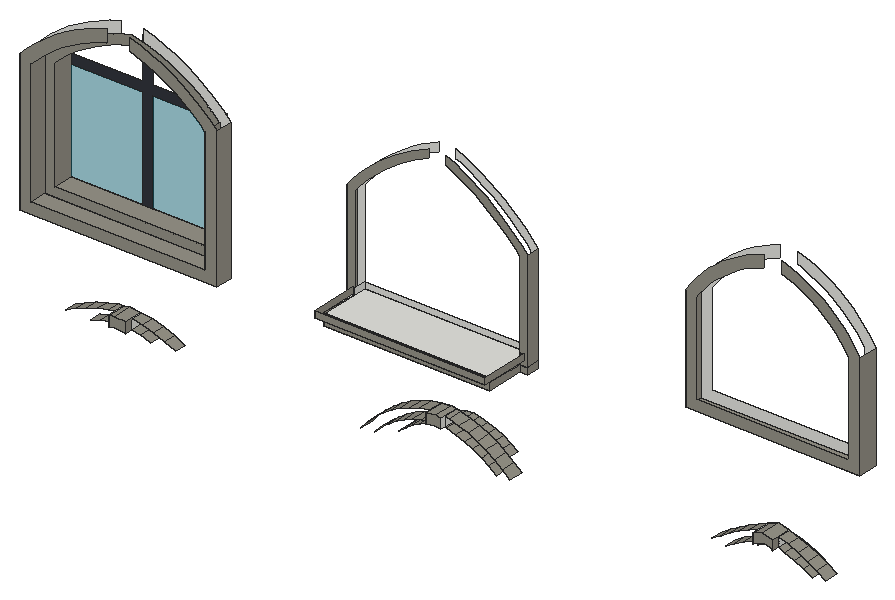
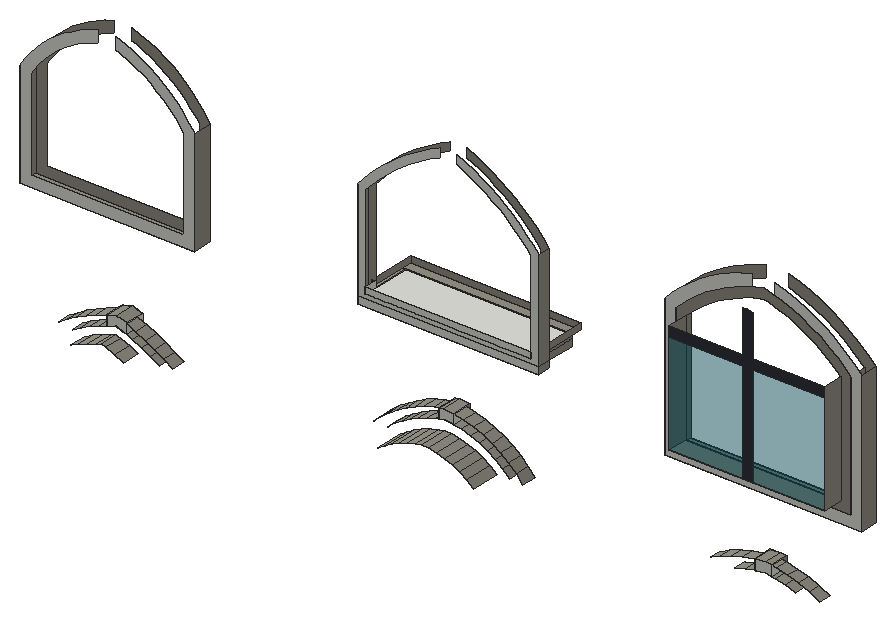
# SketchUp Ruby script. Lengths in inches.
U = 1.inch
M = Sketchup.active_model
def pt(a) = Geom::Point3d.new(a.map { |v| v * U })
def face(e, loops, mat)
  f = e.add_face(loops[0].map { |a| pt(a) })
  loops[1..].each { |l| e.add_face(l.map { |a| pt(a) }).erase! }
  f.material = f.back_material = mat if mat
  f
end
# faces: each face lists its corners as indices into pts; further lists are holes
def faces(e, pts, list, mat = nil) = list.each { |f| face(e, (f[0].is_a?(Array) ? f : [f]).map { |l| l.map { |i| pts[i] } }, mat) }
# xy, xz, yz: faces in a plane at the given z, y or x. An outline is a flat list of corners, or four numbers for a rectangle; further outlines are holes
def ring(l) = l.size == 4 ? [[l[0], l[1]], [l[2], l[1]], [l[2], l[3]], [l[0], l[3]]] : l.each_slice(2).to_a
def flat(e, list, mat, &to3) = list.each { |f| face(e, (f[0].is_a?(Array) ? f : [f]).map { |l| ring(l).map { |u, v| to3.(u, v) } }, mat) }
def xy(e, z, list, mat = nil) = flat(e, list, mat) { |x, y| [x, y, z] }
def xz(e, y, list, mat = nil) = flat(e, list, mat) { |x, z| [x, y, z] }
def yz(e, x, list, mat = nil) = flat(e, list, mat) { |y, z| [x, y, z] }
def lines(e, pts, list) = list.each { |a, b| e.add_line(pt(pts[a]), pt(pts[b])) }
# prism: a flat outline (further loops are holes) pulled along v
def prism(e, loops, v, mat = nil)
  f = face(e, loops, mat); d = Geom::Vector3d.new(v.map { |x| x * U })
  f.pushpull(f.normal.samedirection?(d) ? d.length : -d.length)
end
def box(e, o, s, mat = nil) = prism(e, [[o, [o[0] + s[0], o[1], o[2]], [o[0] + s[0], o[1] + s[1], o[2]], [o[0], o[1] + s[1], o[2]]]], [0, 0, s[2]], mat)
def at(x, y, z, deg = 0) = Geom::Transformation.translation(pt([x, y, z])) * Geom::Transformation.rotation(ORIGIN, Z_AXIS, deg.degrees)
def axes(o, x, y, z) = Geom::Transformation.new([*x, 0, *y, 0, *z, 0, *pt(o).to_a, 1])
def part(name) = M.definitions.add(name)
# library, detail: a bought-in or finely detailed component or shape, given as its bounding box
def library(name, o, s) = part(name).tap { |d| box(d.entities, o, s) }
def detail(e, o, s) = box(e.add_group.entities, o, s)
def put(e, d, t, mat = nil) = e.add_instance(d, t).tap { |i| i.material = mat if mat }
def group(e, t, mat = nil) = e.add_group.tap { |g| g.transformation = t; g.material = mat if mat }.entities
root = M.entities
M.materials.add("[Formica Graystone]").color = [149, 146, 135]
M.materials.add("[Formica Laminate Dark]").color = [50, 53, 60]
M.materials.add("[Translucent Glass Tinted]").color = [4, 106, 127]
M.materials["[Translucent Glass Tinted]"].alpha = 0.48
xy(root,431.0625,[[55.73,135.41,152.02,144.04]],"[Formica Graystone]")
xy(root,436.63,[[61.3,135.41,146.45,144.04]],"[Formica Graystone]")
xy(root,441.07,[[65.73,144.04,142.02,154.22]],"[Formica Graystone]")
xy(root,444.43,[[217.65,119.16,217.65,137.66,213.87,137.66,213.87,144.04,302.49,144.04,302.49,137.66,298.71,137.66,298.71,119.16]],"[Formica Graystone]")
xy(root,447.8,[[217.65,119.16,298.71,119.16,298.71,137.66,302.49,137.66,302.49,144.04,213.87,144.04,213.87,137.66,217.65,137.66]])
xy(root,449.51,[[370.76,148.68,456.27,158.3]],"[Formica Graystone]")
xy(root,449.83,[[216.84,119.16,217.65,137.66],[217.65,119.16,298.71,144.04]])
xy(root,449.83,[[216.84,114.16,300.34,119.16],[298.71,119.16,300.34,137.66]],"[Formica Graystone]")
xz(root,114.16,[[216.84,449.83,300.34,452.9]],"[Formica Graystone]")
xz(root,119.16,[[217.65,444.43,298.71,447.8],[217.65,447.8,298.71,449.83]],"[Formica Graystone]")
xz(root,134.29,[[262.44,408.08,262.44,412.87,260.05,413.37,255.1,412.87,255.1,408.09,255.79,408.23,259.8,408.63]],"[Formica Graystone]")
xz(root,134.6,[[108.25,395.78,108.25,400.8125,102.66,401.34,99.89,400.96,99.89,395.97,102.76,396.35,107.57,395.9]],"[Formica Graystone]")
xz(root,135.41,[[55.73,431.0625,152.02,431.0625,152.02,499.53,148.09,503.55,143.91,507.3,139.5,510.79,134.89,513.99,130.08,516.9,125.1,519.51,119.96,521.79,114.7,523.75,109.32,525.375,109.32,519.5625,112.92,518.47,117.86,516.64,122.67,514.49,127.35,512.05,131.85,509.32,136.18,506.32,140.32,503.05,144.23,499.52,146.45,497.26,146.45,436.63,61.3,436.63,61.3,497.1875,63.52,499.43,67.45,502.9375,71.59,506.2,75.92,509.2,80.43,511.9375,85.1,514.39,89.91,516.55,94.84,518.41,98.39,519.51,98.39,525.34,93.03,523.68,87.78,521.7,82.66,519.4,77.69,516.79,72.89,513.875,68.28,510.68,63.87,507.2,59.68,503.46,55.73,499.48]],"[Formica Graystone]")
xz(root,137.66,[[216.84,449.83,217.65,452.9],[298.71,449.83,300.34,452.9]])
xz(root,137.66,[[213.87,444.43,217.65,447.8],[298.71,444.43,302.49,447.8],[213.87,447.8,217.65,447.8,217.65,449.83,216.84,449.83,216.84,452.9,217.65,452.9,217.65,495.41,219.67,497.78,222.68,501.01,225.83,504.11,229.125,507.06,232.54,509.86,236.08,512.5,239.74,514.99,243.5,517.3,247.37,519.45,251.32,521.42,253.91,522.5625,253.91,526.7,249.71,524.84,245.6,522.8,241.59,520.57,237.68,518.16,233.89,515.59,230.21,512.84,226.66,509.93,223.25,506.87,219.97,503.65,216.84,500.3,213.87,496.8],[298.71,447.8,302.49,447.8,302.49,496.8,299.44,500.21,296.25,503.5,292.9375,506.65,289.49,509.67,285.93,512.55,282.26,515.28,278.48,517.86,274.59,520.28,270.62,522.55,266.55,524.66,262.4,526.6,262.4,522.42,264.88,521.26,268.81,519.23,272.65,517.04,276.41,514.69,280.0625,512.2,283.61,509.56,287.06,506.78,290.38,503.86,293.59,500.81,296.67,497.63,298.71,495.36,298.71,452.9,300.34,452.9,300.34,449.83,298.71,449.83]],"[Formica Graystone]")
xz(root,144.04,[[108.25,395.78,107.57,395.9,102.76,396.35,99.89,395.97,99.89,400.96,102.66,401.34,108.25,400.8125],[262.44,408.08,259.8,408.63,255.79,408.23,255.1,408.09,255.1,412.87,260.05,413.37,262.44,412.87],[55.73,431.0625,55.73,499.48,59.68,503.46,63.87,507.2,68.28,510.68,72.89,513.875,77.69,516.79,82.66,519.4,87.78,521.7,93.03,523.68,98.39,525.34,98.39,519.51,94.84,518.41,89.91,516.55,85.1,514.39,80.43,511.9375,75.92,509.2,71.59,506.2,67.45,502.9375,63.52,499.43,61.3,497.1875,61.3,436.63,146.45,436.63,146.45,497.26,144.23,499.52,140.32,503.05,136.18,506.32,131.85,509.32,127.35,512.05,122.67,514.49,117.86,516.64,112.92,518.47,109.32,519.5625,109.32,525.375,114.7,523.75,119.96,521.79,125.1,519.51,130.08,516.9,134.89,513.99,139.5,510.79,143.91,507.3,148.09,503.55,152.02,499.53,152.02,431.0625],[213.87,444.43,302.49,447.8],[213.87,447.8,213.87,496.8,216.84,500.3,219.97,503.65,223.25,506.87,226.66,509.93,230.21,512.84,233.89,515.59,237.68,518.16,241.59,520.57,245.6,522.8,249.71,524.84,253.91,526.7,253.91,522.5625,251.32,521.42,247.37,519.45,243.5,517.3,239.74,514.99,236.08,512.5,232.54,509.86,229.125,507.06,225.83,504.11,222.68,501.01,219.67,497.78,217.65,495.41,217.65,449.83,298.71,449.83,298.71,495.36,296.67,497.63,293.59,500.81,290.38,503.86,287.06,506.78,283.61,509.56,280.0625,512.2,276.41,514.69,272.65,517.04,268.81,519.23,264.88,521.26,262.4,522.42,262.4,526.6,266.55,524.66,270.62,522.55,274.59,520.28,278.48,517.86,282.26,515.28,285.93,512.55,289.49,509.67,292.9375,506.65,296.25,503.5,299.44,500.21,302.49,496.8,302.49,447.8],
  [217.65,449.83,298.71,452.9]])
xz(root,144.04,[[[61.3,436.63,146.45,436.63,146.45,497.26,144.23,499.52,140.32,503.05,136.18,506.32,131.85,509.32,127.35,512.05,122.67,514.49,117.86,516.64,112.92,518.47,109.32,519.5625,107.875,520,103.87,520.9375,99.875,519.97,98.39,519.51,94.84,518.41,89.91,516.55,85.1,514.39,80.43,511.9375,75.92,509.2,71.59,506.2,67.45,502.9375,63.52,499.43,61.3,497.1875],[65.73,441.07,65.73,495.36,66.57,496.21,70.3,499.54,74.23,502.63,78.34,505.48,82.61,508.07,87.04,510.4,91.6,512.45,96.28,514.21,101.05,515.6875,103.89,516.375,106.73,515.71,111.5,514.27,116.18,512.53,120.74,510.5,125.17,508.18,129.4375,505.6,133.54,502.75,137.45,499.65,141.16,496.32,142.02,495.45,142.02,441.07]]],"[Formica Graystone]")
xz(root,148.55,[[404.07,401.49,405.7,402.17,409.0625,403.41,412.52,402.41,413.875,401.94,413.875,406.64,408.9,408.09,404.07,406.31]],"[Formica Graystone]")
xz(root,148.68,[[370.76,449.51,456.27,449.51,456.27,500.95,453.8,504.68,451.07,508.24,448.12,511.6,444.94,514.76,441.56,517.7,437.99,520.4,434.24,522.86,430.34,525.06,426.29,526.99,422.13,528.65,417.87,530.02,417.87,524.45,420.34,523.66,424.17,522.13,427.89,520.36,431.48,518.33,434.93,516.07,438.22,513.58,441.33,510.88,444.25,507.97,446.98,504.875,449.48,501.6,450.98,499.35,450.98,454.81,376.06,454.81,376.06,499.26,377.57,501.39,380.16,504.61,382.95,507.66,385.92,510.53,389.0625,513.22,392.36,515.7,395.8125,517.98,399.4,520.04,403.1,521.87,406.91,523.47,409.22,524.28,409.22,529.89,405.01,528.42,400.9,526.69,396.9,524.71,393.03,522.49,389.31,520.03,385.74,517.35,382.35,514.45,379.15,511.35,376.14,508.06,373.34,504.58,370.76,500.95]],"[Formica Graystone]")
xz(root,154.22,[[101.05,441.07,105.93,441.07,105.93,490.64,142.02,490.64,142.02,495.36,105.93,495.36,105.93,515.9,103.89,516.375,101.05,515.6875,101.05,495.36,65.73,495.36,65.73,490.64,101.05,490.64]],"[Formica Laminate Dark]")
xz(root,154.22,[[65.73,441.07,101.05,490.64],[105.93,441.07,142.02,490.64]],"[Translucent Glass Tinted]")
xz(root,158.3,[[404.07,401.49,404.07,406.31,408.9,408.09,413.875,406.64,413.875,401.94,412.52,402.41,409.0625,403.41,405.7,402.17],[370.76,449.51,370.76,500.95,373.34,504.58,376.14,508.06,379.15,511.35,382.35,514.45,385.74,517.35,389.31,520.03,393.03,522.49,396.9,524.71,400.9,526.69,405.01,528.42,409.22,529.89,409.22,524.28,406.91,523.47,403.1,521.87,399.4,520.04,395.8125,517.98,392.36,515.7,389.0625,513.22,385.92,510.53,382.95,507.66,380.16,504.61,377.57,501.39,376.06,499.26,376.06,454.81,450.98,454.81,450.98,499.35,449.48,501.6,446.98,504.875,444.25,507.97,441.33,510.88,438.22,513.58,434.93,516.07,431.48,518.33,427.89,520.36,424.17,522.13,420.34,523.66,417.87,524.45,417.87,530.02,422.13,528.65,426.29,526.99,430.34,525.06,434.24,522.86,437.99,520.4,441.56,517.7,444.94,514.76,448.12,511.6,451.07,508.24,453.8,504.68,456.27,500.95,456.27,449.51]])
yz(root,55.73,[[135.41,431.0625,144.04,499.48]],"[Formica Graystone]")
yz(root,61.3,[[135.41,436.63,144.04,497.1875]],"[Formica Graystone]")
yz(root,65.73,[[144.04,441.07,154.22,495.36]],"[Formica Graystone]")
yz(root,99.89,[[138.29,395.97,144.04,400.96]])
yz(root,99.89,[[134.6,395.97,138.29,400.96]],"[Formica Graystone]")
yz(root,108.25,[[138.29,395.78,144.04,400.8125]])
yz(root,108.25,[[134.6,395.78,138.29,400.8125]],"[Formica Graystone]")
yz(root,142.02,[[144.04,441.07,154.22,495.45]],"[Formica Graystone]")
yz(root,146.45,[[135.41,436.63,144.04,497.26]],"[Formica Graystone]")
yz(root,152.02,[[135.41,431.0625,144.04,499.53]],"[Formica Graystone]")
yz(root,213.87,[[137.66,444.43,144.04,447.8],[137.66,447.8,144.04,496.8]],"[Formica Graystone]")
yz(root,216.84,[[114.16,449.83,137.66,452.9]],"[Formica Graystone]")
yz(root,217.65,[[137.66,449.83,144.04,452.9]])
yz(root,217.65,[[119.16,444.43,137.66,447.8],[119.16,447.8,137.66,449.83]],"[Formica Graystone]")
yz(root,255.1,[[136.91,408.09,144.04,412.87]])
yz(root,255.1,[[134.29,408.09,136.91,412.87]],"[Formica Graystone]")
yz(root,262.44,[[134.29,408.08,136.91,412.87],[136.91,408.08,144.04,412.87]])
yz(root,298.71,[[137.66,449.83,144.04,452.9]])
yz(root,298.71,[[119.16,444.43,137.66,447.8],[119.16,447.8,137.66,449.83]],"[Formica Graystone]")
yz(root,300.34,[[114.16,449.83,137.66,452.9]],"[Formica Graystone]")
yz(root,302.49,[[137.66,444.43,144.04,447.8],[137.66,447.8,144.04,496.8]],"[Formica Graystone]")
yz(root,370.76,[[148.68,449.51,158.3,500.95]],"[Formica Graystone]")
yz(root,404.07,[[148.55,401.49,151.8,406.31],[151.8,401.49,158.3,406.31]])
yz(root,413.875,[[151.8,401.94,158.3,406.64]])
yz(root,413.875,[[148.55,401.94,151.8,406.64]],"[Formica Graystone]")
yz(root,456.27,[[148.68,449.51,158.3,500.95]],"[Formica Graystone]")
p = [[87.98,144.04,393.1],[92.93,144.04,394.6],[92.93,138.29,394.6],[87.98,138.29,393.1],[224.71,144.04,397.08],[221.45,144.04,393.3125],
  [221.45,136.91,393.3125],[224.71,136.91,397.08],[81.15,144.04,395.73],[76.15,144.04,393.27],[76.15,138.29,393.27],[81.15,138.29,395.73],
  [237.6875,144.04,395.96],[234.47,144.04,393.42],[234.47,158.1,393.42],[237.6875,158.1,395.96],[387.95,158.3,393.39],[392.24,158.3,395.87],
  [392.24,151.8,395.87],[387.95,151.8,393.39],[424.4375,158.3,393.36],[420.18,158.3,395.41],[420.18,167.05,395.41],[424.4375,167.05,393.36],
  [112.67,144.04,394.96],[117.67,144.04,393.58],[117.67,138.29,393.58],[112.67,138.29,394.96],[228.11,144.04,393.84],[231.39,144.04,396.98],
  [231.39,136.91,396.98],[228.11,136.91,393.84],[129.53,144.04,393.91],[124.46,144.04,396.33],[124.46,138.29,396.33],[129.53,138.29,393.91],
  [385.65,158.3,397.19],[381.31,158.3,394.4375],[381.31,151.8,394.4375],[385.65,151.8,397.19],[426.18,158.3,396.74],[430.51,158.3,394.36],
  [430.51,151.8,394.36],[426.18,151.8,396.74],[281.4,144.04,394.54],[277.91,144.04,396.84],[277.91,158.1,396.84],[281.4,158.1,394.54],
  [97.99,144.04,395.71],[97.99,138.29,395.71],[402.67,158.3,396.78],[398.33,158.3,394.75],[398.33,167.05,394.75],[402.67,167.05,396.78],
  [108.25,144.04,395.78],[108.25,138.29,395.78],[437.15,158.3,395.44],[432.76,158.3,398.19],[432.76,151.8,398.19],[437.15,151.8,395.44],
  [415.8125,158.3,397.22],[415.8125,167.05,397.22],[284.14,144.04,398.37],[287.72,144.04,395.59],[287.72,136.91,395.59],[284.14,136.91,398.37],
  [86.34,144.04,397.78],[86.34,138.29,397.78],[99.89,144.04,395.97],[99.89,138.29,395.97],[107.57,144.04,395.9],[108.25,134.6,395.78],
  [107.57,134.6,395.9],[102.76,144.04,396.35],[102.76,134.6,396.35],[294.35,144.04,395.92],[290.73,144.04,399.19],[290.73,136.91,399.19],
  [294.35,136.91,395.92],[396.64,158.3,398.16],[396.64,151.8,398.16],[99.89,134.6,395.97],[241.125,144.04,398.18],[241.125,158.1,398.18],
  [119.2,144.04,398.3],[119.2,138.29,398.3],[421.74,158.3,398.88],[421.74,151.8,398.88],[274.27,144.04,398.875],[274.27,158.1,398.875],
  [407.09,158.3,398.63],[407.09,167.05,398.63],[234.95,144.04,399.79],[234.95,136.91,399.79],[228.31,144.04,400.52],[228.31,136.91,400.52],
  [390.1,158.3,399.77],[390.1,151.8,399.77],[411.36,158.3,398.78],[411.36,167.05,398.78],[91.68,144.04,399.4],[91.68,138.29,399.4],
  [244.76,144.04,400.07],[244.76,158.1,400.07],[401.12,158.3,400.26],[401.12,151.8,400.26],[428.22,158.3,400.69],[428.22,151.8,400.69],
  [113.78,144.04,399.8],[113.78,138.29,399.8],[280.36,144.04,400.86],[280.36,136.91,400.86],[409.2,158.3,399.41],[409.2,167.05,399.41],
  [270.47,144.04,400.625],[270.47,158.1,400.625],[417.18,158.3,400.78],[417.18,151.8,400.78],[286.86,144.04,402.18],[286.86,136.91,402.18],
  [97.13,144.04,400.59],[97.13,138.29,400.59],[238.76,144.04,402.25],[238.76,136.91,402.25],[108.25,144.04,400.8125],[108.25,138.29,400.8125],
  [394.66,158.3,402.14],[394.66,151.8,402.14],[248.55,144.04,401.61],[248.55,158.1,401.61],[404.07,158.3,401.49],[404.07,151.8,401.49],
  [232.22,144.04,403.6],[232.22,136.91,403.6],[99.89,144.04,400.96],[99.89,138.29,400.96],[266.5625,144.04,402.09],[266.5625,158.1,402.09],
  [423.55,158.3,402.94],[423.55,151.8,402.94],[102.66,144.04,401.34],[102.66,134.6,401.34],[108.25,134.6,400.8125],[413.875,158.3,401.94],
  [413.875,151.8,401.94],[276.4,144.04,403.07],[276.4,136.91,403.07],[99.89,134.6,400.96],[405.7,158.3,402.17],[405.7,148.55,402.17],
  [404.07,148.55,401.49],[252.47,144.04,402.78],[252.47,158.1,402.78],[412.52,158.3,402.41],[413.875,148.55,401.94],[412.52,148.55,402.41],
  [262.55,144.04,403.25],[262.55,158.1,403.25],[399.32,158.3,404.33],[399.32,151.8,404.33],[282.79,144.04,404.87],[282.79,136.91,404.87],
  [409.0625,158.3,403.41],[409.0625,148.55,403.41],[242.79,144.04,404.34],[242.79,136.91,404.34],[256.49,144.04,403.57],[256.49,158.1,403.57],
  [418.76,158.3,404.93],[418.76,151.8,404.93],[272.29,144.04,404.97],[272.29,136.91,404.97],[259.55,144.04,403.88],[259.55,158.1,403.88],
  [260.1,158.1,403.77],[236.4,144.04,406.31],[236.4,136.91,406.31],[246.99,144.04,406.05],[246.99,136.91,406.05],[404.07,158.3,406.31],
  [404.07,151.8,406.31],[278.52,144.04,407.25],[278.52,136.91,407.25],[413.875,158.3,406.64],[413.875,151.8,406.64],[268.04,144.04,406.55],
  [268.04,136.91,406.55],[251.34,144.04,407.34],[251.34,136.91,407.34],[240.82,144.04,408.6],[240.82,136.91,408.6],[408.9,158.3,408.09],
  [404.07,148.55,406.31],[408.9,148.55,408.09],[263.69,144.04,407.82],[263.69,136.91,407.82],[413.875,148.55,406.64],[274.09,144.04,409.29],
  [274.09,136.91,409.29],[255.1,144.04,408.09],[255.1,136.91,408.09],[262.44,144.04,408.08],[262.44,136.91,408.08],[255.79,144.04,408.23],
  [255.79,134.29,408.23],[255.1,134.29,408.09],[259.8,144.04,408.63],[262.44,134.29,408.08],[259.8,134.29,408.63],[245.4375,144.04,410.47],
  [245.4375,136.91,410.47],[269.52,144.04,411],[269.52,136.91,411],[250.21,144.04,411.9],[250.21,136.91,411.9],[264.83,144.04,412.37],
  [264.83,136.91,412.37],[255.1,144.04,412.87],[255.1,136.91,412.87],[262.44,144.04,412.87],[262.44,136.91,412.87],[260.05,144.04,413.37],
  [255.1,134.29,412.87],[260.05,134.29,413.37],[262.44,134.29,412.87]]
faces(root,p,[[0,1,2,3],[4,5,6,7],[8,9,10,11],[12,13,14,15],[16,17,18,19],[20,21,22,23],[24,25,26,27],[28,29,30,31],
  [32,33,34,35],[36,37,38,39],[40,41,42,43],[44,45,46,47],[1,48,49,2],[50,51,52,53],[54,24,27,55],[56,57,58,59],
  [21,60,61,22],[62,63,64,65],[66,8,11,67],[48,68,69,49],[70,54,55,71,72],[73,70,72,74],[75,76,77,78],[17,79,80,18],
  [68,73,74,81,69],[82,12,15,83],[33,84,85,34],[86,40,43,87],[45,88,89,46],[90,50,53,91],[29,92,93,30],[94,4,7,95],
  [96,36,39,97],[60,98,99,61],[100,66,67,101],[102,82,83,103],[79,104,105,80],[57,106,107,58],[84,108,109,85],[110,62,65,111],
  [112,90,91,113],[98,112,113,99],[88,114,115,89],[116,86,87,117],[76,118,119,77],[120,100,101,121],[92,122,123,93],[108,124,125,109],
  [126,96,97,127],[128,102,103,129],[104,130,131,105],[132,94,95,133],[134,120,121,135],[114,136,137,115],[106,138,139,107],[124,140,141,142,125],
  [143,116,117,144],[145,110,111,146],[140,134,135,147,141],[130,148,149,150,131],[151,128,129,152],[153,143,144,154,155],[136,156,157,137],[158,126,127,159],
  [118,160,161,119],[148,162,163,149],[122,164,165,123],[162,153,155,163],[166,151,152,167],[138,168,169,139],[170,145,146,171],[156,172,173,174,157],
  [175,132,133,176],[172,166,167,173],[164,177,178,165],[179,158,159,180],[160,181,182,161],[168,183,184,169],[185,170,171,186],[177,187,188,178],
  [189,175,176,190],[191,179,180,192,193],[194,185,186,195],[183,191,193,196,184],[181,197,198,182],[187,199,200,188],[201,194,195,202],[199,203,204,205,200],
  [206,201,202,207,208],[203,206,208,204],[209,189,190,210],[197,211,212,198],[213,209,210,214],[211,215,216,212],[217,213,214,218],[215,219,220,216],
  [221,217,218,222,223],[219,221,223,224,220]],"[Formica Graystone]")
